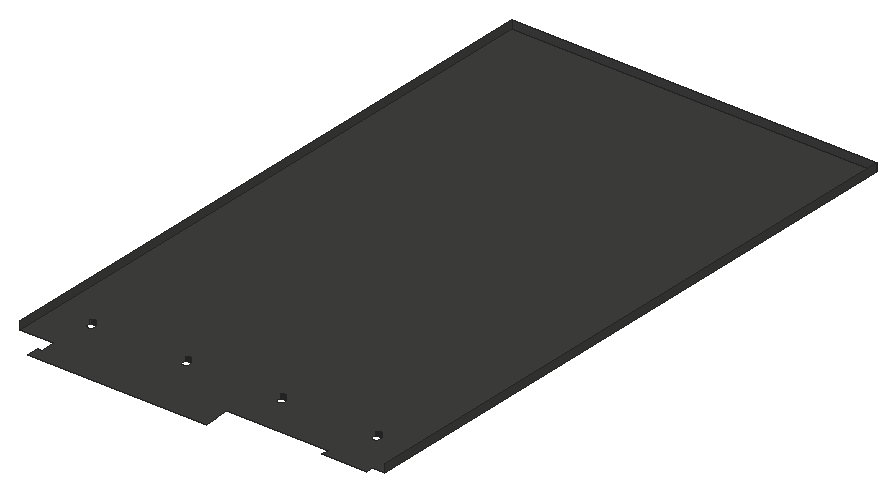
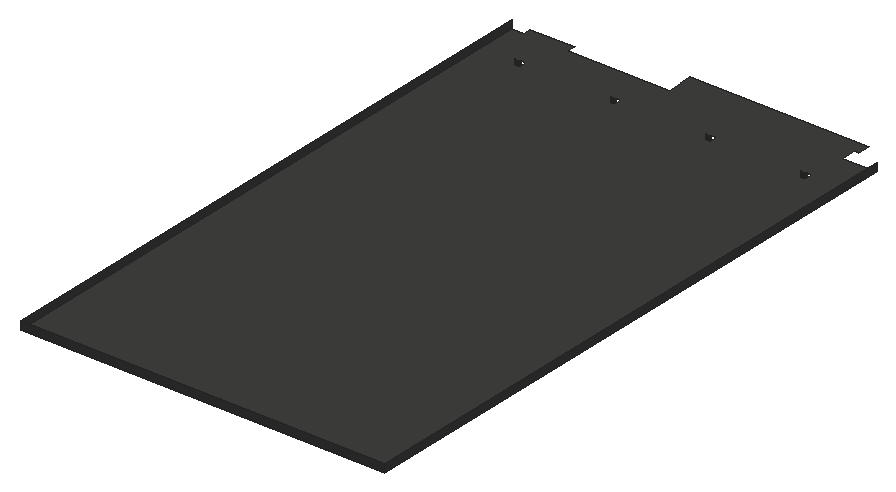
# SketchUp Ruby script. Lengths in inches.
U = 1.inch
M = Sketchup.active_model
def pt(a) = Geom::Point3d.new(a.map { |v| v * U })
def face(e, loops, mat)
  f = e.add_face(loops[0].map { |a| pt(a) })
  loops[1..].each { |l| e.add_face(l.map { |a| pt(a) }).erase! }
  f.material = f.back_material = mat if mat
  f
end
# faces: each face lists its corners as indices into pts; further lists are holes
def faces(e, pts, list, mat = nil) = list.each { |f| face(e, (f[0].is_a?(Array) ? f : [f]).map { |l| l.map { |i| pts[i] } }, mat) }
# xy, xz, yz: faces in a plane at the given z, y or x. An outline is a flat list of corners, or four numbers for a rectangle; further outlines are holes
def ring(l) = l.size == 4 ? [[l[0], l[1]], [l[2], l[1]], [l[2], l[3]], [l[0], l[3]]] : l.each_slice(2).to_a
def flat(e, list, mat, &to3) = list.each { |f| face(e, (f[0].is_a?(Array) ? f : [f]).map { |l| ring(l).map { |u, v| to3.(u, v) } }, mat) }
def xy(e, z, list, mat = nil) = flat(e, list, mat) { |x, y| [x, y, z] }
def xz(e, y, list, mat = nil) = flat(e, list, mat) { |x, z| [x, y, z] }
def yz(e, x, list, mat = nil) = flat(e, list, mat) { |y, z| [x, y, z] }
def lines(e, pts, list) = list.each { |a, b| e.add_line(pt(pts[a]), pt(pts[b])) }
# prism: a flat outline (further loops are holes) pulled along v
def prism(e, loops, v, mat = nil)
  f = face(e, loops, mat); d = Geom::Vector3d.new(v.map { |x| x * U })
  f.pushpull(f.normal.samedirection?(d) ? d.length : -d.length)
end
def box(e, o, s, mat = nil) = prism(e, [[o, [o[0] + s[0], o[1], o[2]], [o[0] + s[0], o[1] + s[1], o[2]], [o[0], o[1] + s[1], o[2]]]], [0, 0, s[2]], mat)
def at(x, y, z, deg = 0) = Geom::Transformation.translation(pt([x, y, z])) * Geom::Transformation.rotation(ORIGIN, Z_AXIS, deg.degrees)
def axes(o, x, y, z) = Geom::Transformation.new([*x, 0, *y, 0, *z, 0, *pt(o).to_a, 1])
def part(name) = M.definitions.add(name)
# library, detail: a bought-in or finely detailed component or shape, given as its bounding box
def library(name, o, s) = part(name).tap { |d| box(d.entities, o, s) }
def detail(e, o, s) = box(e.add_group.entities, o, s)
def put(e, d, t, mat = nil) = e.add_instance(d, t).tap { |i| i.material = mat if mat }
def group(e, t, mat = nil) = e.add_group.tap { |g| g.transformation = t; g.material = mat if mat }.entities
root = M.entities
M.materials.add("1448 AP 8253 RAVEN SONG").color = [64, 64, 63]
xy(root,372,[[[31.93,174,31.93,183,35.02,183,35.02,195,9.27,195,9.27,663,287.37,663,287.37,195,278.1,195,278.1,189,244.11,189,244.11,195,166.86,195,166.86,183,167.89,183,167.89,174],[257.03,221.5,257.35,221.5,257.43,221.51,257.5,221.52,257.74,221.55,257.8125,221.57,257.89,221.58,257.97,221.6,258.04,221.625,258.12,221.65,258.19,221.67,258.27,221.7,258.48,221.79,258.55,221.83,258.62,221.86,258.76,221.94,258.82,221.98,258.89,222.03,258.95,222.07,259.02,222.12,259.26,222.32,259.3125,222.38,259.37,222.43,259.57,222.67,259.62,222.74,259.66,222.8,259.71,222.87,259.75,222.93,259.83,223.07,259.86,223.14,259.9,223.21,259.99,223.42,260.02,223.5,260.04,223.57,260.07,223.65,260.09,223.72,260.11,223.8,260.14,223.95,260.16,224.11,260.17,224.1875,260.18,224.26,260.1875,224.34,260.1875,224.42,260.19,224.5,260.1875,224.58,260.1875,224.66,260.18,224.74,260.17,224.8125,260.16,224.89,260.14,225.05,260.11,225.2,260.09,225.28,260.07,225.35,260.04,225.43,260.02,225.5,259.99,225.58,259.9,225.79,259.86,225.86,259.83,225.93,259.75,226.07,259.71,226.13,259.66,226.2,259.62,226.26,259.57,226.33,259.37,226.57,259.3125,226.62,259.26,226.68,259.02,226.88,258.95,226.93,258.89,226.97,258.82,227.02,258.76,227.06,258.62,227.14,258.55,227.17,258.48,227.21,258.27,227.3,258.19,227.33,258.12,227.35,258.04,227.375,257.97,227.4,257.89,227.42,257.8125,227.43,257.74,227.45,257.5,227.48,257.43,227.49,257.35,227.5,257.03,227.5,256.95,227.49,256.8,227.47,256.64,227.45,256.57,227.43,256.49,227.42,256.41,227.4,256.34,227.375,256.26,227.35,256.1875,227.33,256.11,227.3,255.9,227.21,255.83,227.17,255.76,227.14,255.62,227.06,255.56,227.02,255.49,226.97,255.43,226.93,255.36,226.88,255.18,226.73,255.125,226.68,255.07,226.62,255.01,226.57,254.81,226.33,254.76,226.26,254.72,226.2,254.67,226.13,254.63,226.07,254.55,225.93,254.52,225.86,254.48,225.79,254.39,225.58,254.36,225.5,254.34,225.43,254.3125,225.35,254.29,225.28,254.27,225.2,254.26,225.125,254.24,225.05,254.22,224.89,254.21,224.8125,254.2,224.74,254.19,224.66,254.19,224.34,254.2,224.26,254.21,224.1875,254.22,224.11,254.24,223.95,254.26,223.875,254.27,223.8,254.29,223.72,254.3125,223.65,254.34,223.57,254.36,223.5,254.39,223.42,254.48,223.21,254.52,223.14,254.55,223.07,254.63,222.93,254.67,222.87,254.72,222.8,254.76,222.74,254.81,222.67,255.01,222.43,255.07,222.38,255.125,222.32,255.18,222.27,255.36,222.12,255.43,222.07,255.49,222.03,255.56,221.98,255.62,221.94,255.76,221.86,255.83,221.83,255.9,221.79,256.11,221.7,256.1875,221.67,256.26,221.65,256.34,221.625,256.41,221.6,256.49,221.58,256.57,221.57,256.64,221.55,256.8,221.53,256.95,221.51],[184.45,221.5,184.77,221.5,184.85,221.51,184.92,221.52,185.16,221.55,185.23,221.57,185.31,221.58,185.39,221.6,185.46,221.625,185.54,221.65,185.61,221.67,185.69,221.7,185.9,221.79,185.97,221.83,186.04,221.86,186.18,221.94,186.24,221.98,186.31,222.03,186.375,222.07,186.5,222.17,186.68,222.32,186.73,222.38,186.79,222.43,186.99,222.67,187.04,222.74,187.08,222.8,187.125,222.87,187.17,222.93,187.25,223.07,187.28,223.14,187.32,223.21,187.41,223.42,187.4375,223.5,187.46,223.57,187.49,223.65,187.51,223.72,187.53,223.8,187.54,223.875,187.56,223.95,187.58,224.11,187.59,224.1875,187.6,224.26,187.61,224.34,187.61,224.66,187.6,224.74,187.59,224.8125,187.58,224.89,187.56,225.05,187.54,225.125,187.53,225.2,187.51,225.28,187.49,225.35,187.46,225.43,187.4375,225.5,187.41,225.58,187.32,225.79,187.28,225.86,187.25,225.93,187.17,226.07,187.125,226.13,187.08,226.2,187.04,226.26,186.99,226.33,186.79,226.57,186.73,226.62,186.68,226.68,186.5,226.83,186.375,226.93,186.31,226.97,186.24,227.02,186.18,227.06,186.04,227.14,185.97,227.17,185.9,227.21,185.69,227.3,185.61,227.33,185.54,227.35,185.46,227.375,185.39,227.4,185.31,227.42,185.23,227.43,185.16,227.45,184.92,227.48,184.85,227.49,184.77,227.5,184.45,227.5,184.3,227.48,184.14,227.46,184.0625,227.45,183.99,227.43,183.91,227.42,183.83,227.4,183.76,227.375,183.68,227.35,183.61,227.33,183.53,227.3,183.32,227.21,183.25,227.17,183.18,227.14,183.04,227.06,182.98,227.02,182.91,226.97,182.85,226.93,182.78,226.88,182.54,226.68,182.49,226.62,182.43,226.57,182.23,226.33,182.18,226.26,182.14,226.2,182.09,226.13,182.05,226.07,181.97,225.93,181.9375,225.86,181.9,225.79,181.81,225.58,181.78,225.5,181.76,225.43,181.73,225.35,181.71,225.28,181.69,225.2,181.68,225.125,181.66,225.05,181.64,224.89,181.625,224.8125,181.62,224.74,181.61,224.66,181.61,224.34,181.62,224.26,181.625,224.1875,181.64,224.11,181.66,223.95,181.68,223.875,181.69,223.8,181.71,223.72,181.73,223.65,181.76,223.57,181.78,223.5,181.81,223.42,181.9,223.21,181.9375,223.14,181.97,223.07,182.05,222.93,182.09,222.87,182.14,222.8,182.18,222.74,182.23,222.67,182.43,222.43,182.49,222.38,182.54,222.32,182.78,222.12,182.85,222.07,182.91,222.03,182.98,221.98,183.04,221.94,183.18,221.86,183.25,221.83,183.32,221.79,183.53,221.7,183.61,221.67,183.68,221.65,183.76,221.625,183.83,221.6,183.91,221.58,183.99,221.57,184.0625,221.55,184.14,221.54,184.3,221.52],[39.29,221.5,39.61,221.5,39.69,221.51,39.76,221.52,40,221.55,40.07,221.57,40.15,221.58,40.23,221.6,40.3,221.625,40.38,221.65,40.45,221.67,40.53,221.7,40.74,221.79,40.8125,221.83,40.88,221.86,41.02,221.94,41.08,221.98,41.15,222.03,41.21,222.07,41.28,222.12,41.52,222.32,41.57,222.38,41.625,222.43,41.68,222.49,41.83,222.67,41.88,222.74,41.92,222.8,41.97,222.87,42.01,222.93,42.09,223.07,42.16,223.21,42.25,223.42,42.28,223.5,42.3,223.57,42.33,223.65,42.35,223.72,42.37,223.8,42.38,223.875,42.4,223.95,42.42,224.11,42.43,224.1875,42.44,224.26,42.45,224.34,42.45,224.66,42.44,224.74,42.43,224.8125,42.42,224.89,42.4,225.05,42.38,225.125,42.37,225.2,42.35,225.28,42.33,225.35,42.3,225.43,42.28,225.5,42.25,225.58,42.16,225.79,42.09,225.93,42.01,226.07,41.97,226.13,41.92,226.2,41.88,226.26,41.83,226.33,41.68,226.51,41.625,226.57,41.57,226.62,41.52,226.68,41.28,226.88,41.21,226.93,41.15,226.97,41.08,227.02,41.02,227.06,40.88,227.14,40.8125,227.17,40.74,227.21,40.53,227.3,40.45,227.33,40.38,227.35,40.3,227.375,40.23,227.4,40.15,227.42,40.07,227.43,40,227.45,39.76,227.48,39.69,227.49,39.61,227.5,39.29,227.5,39.21,227.49,39.14,227.48,38.9,227.45,38.83,227.43,38.75,227.42,38.67,227.4,38.6,227.375,38.52,227.35,38.45,227.33,38.3,227.27,38.16,227.21,38.09,227.17,38.02,227.14,37.88,227.06,37.82,227.02,37.75,226.97,37.6875,226.93,37.5,226.78,37.38,226.68,37.33,226.62,37.27,226.57,37.07,226.33,37.02,226.26,36.98,226.2,36.93,226.13,36.89,226.07,36.85,226,36.8125,225.93,36.78,225.86,36.74,225.79,36.65,225.58,36.62,225.5,36.6,225.43,36.57,225.35,36.55,225.28,36.53,225.2,36.52,225.125,36.5,225.05,36.48,224.89,36.47,224.8125,36.46,224.74,36.45,224.66,36.45,224.34,36.46,224.26,36.47,224.1875,36.48,224.11,36.5,223.95,36.52,223.875,36.53,223.8,36.55,223.72,36.57,223.65,36.6,223.57,36.62,223.5,36.65,223.42,36.74,223.21,36.78,223.14,36.8125,223.07,36.85,223,36.89,222.93,36.93,222.87,36.98,222.8,37.02,222.74,37.07,222.67,37.27,222.43,37.33,222.38,37.38,222.32,37.5,222.22,37.6875,222.07,37.75,222.03,37.82,221.98,37.88,221.94,38.02,221.86,38.09,221.83,38.16,221.79,38.3,221.73,38.45,221.67,38.52,221.65,38.6,221.625,38.67,221.6,38.75,221.58,38.83,221.57,38.9,221.55,39.14,221.52,39.21,221.51],[111.87,221.5,112.1875,221.5,112.27,221.51,112.34,221.52,112.58,221.55,112.65,221.57,112.73,221.58,112.81,221.6,112.88,221.625,112.96,221.65,113.03,221.67,113.11,221.7,113.32,221.79,113.39,221.83,113.46,221.86,113.6,221.94,113.66,221.98,113.73,222.03,113.79,222.07,113.86,222.12,114.1,222.32,114.15,222.38,114.21,222.43,114.26,222.49,114.3125,222.55,114.36,222.61,114.41,222.67,114.46,222.74,114.5,222.8,114.55,222.87,114.59,222.93,114.67,223.07,114.7,223.14,114.74,223.21,114.83,223.42,114.86,223.5,114.88,223.57,114.91,223.65,114.93,223.72,114.95,223.8,114.96,223.875,114.98,223.95,115,224.11,115.01,224.1875,115.02,224.26,115.03,224.34,115.03,224.66,115.02,224.74,115.01,224.8125,115,224.89,114.98,225.05,114.96,225.125,114.95,225.2,114.93,225.28,114.91,225.35,114.88,225.43,114.86,225.5,114.83,225.58,114.74,225.79,114.7,225.86,114.67,225.93,114.59,226.07,114.55,226.13,114.5,226.2,114.46,226.26,114.41,226.33,114.36,226.39,114.3125,226.45,114.26,226.51,114.21,226.57,114.15,226.62,114.1,226.68,113.86,226.88,113.79,226.93,113.73,226.97,113.66,227.02,113.6,227.06,113.46,227.14,113.39,227.17,113.32,227.21,113.11,227.3,113.03,227.33,112.96,227.35,112.88,227.375,112.81,227.4,112.73,227.42,112.65,227.43,112.58,227.45,112.34,227.48,112.27,227.49,112.1875,227.5,111.87,227.5,111.79,227.49,111.72,227.48,111.64,227.47,111.5625,227.46,111.48,227.45,111.41,227.43,111.33,227.42,111.25,227.4,111.18,227.375,111.1,227.35,111.03,227.33,110.95,227.3,110.74,227.21,110.67,227.17,110.6,227.14,110.46,227.06,110.4,227.02,110.33,226.97,110.27,226.93,110.2,226.88,109.96,226.68,109.91,226.62,109.85,226.57,109.65,226.33,109.6,226.26,109.56,226.2,109.51,226.13,109.47,226.07,109.39,225.93,109.36,225.86,109.32,225.79,109.23,225.58,109.2,225.5,109.18,225.43,109.15,225.35,109.13,225.28,109.11,225.2,109.1,225.125,109.08,225.05,109.06,224.89,109.05,224.8125,109.04,224.74,109.03,224.66,109.03,224.34,109.04,224.26,109.05,224.1875,109.06,224.11,109.08,223.95,109.1,223.875,109.11,223.8,109.13,223.72,109.15,223.65,109.18,223.57,109.2,223.5,109.23,223.42,109.32,223.21,109.36,223.14,109.39,223.07,109.47,222.93,109.51,222.87,109.56,222.8,109.6,222.74,109.65,222.67,109.85,222.43,109.91,222.38,109.96,222.32,110.2,222.12,110.27,222.07,110.33,222.03,110.4,221.98,110.46,221.94,110.6,221.86,110.67,221.83,110.74,221.79,110.95,221.7,111.03,221.67,111.1,221.65,111.18,221.625,111.25,221.6,111.33,221.58,111.41,221.57,111.48,221.55,111.5625,221.54,111.64,221.53,111.72,221.52,111.79,221.51]]],"1448 AP 8253 RAVEN SONG")
xz(root,227.5,[[39.29,372,39.37,375],[39.37,372,39.45,375],[39.45,372,39.53,375],[39.53,372,39.61,375],[111.87,372,111.95,375],
  [111.95,372,112.03,375],[112.03,372,112.11,375],[112.11,372,112.1875,375],[184.45,372,184.53,375],[184.53,372,184.61,375],
  [184.61,372,184.6875,375],[184.6875,372,184.77,375],[257.03,372,257.11,375],[257.11,372,257.19,375],[257.19,372,257.27,375],
  [257.27,372,257.35,375]],"1448 AP 8253 RAVEN SONG")
xz(root,663,[[9.27,372,287.37,378]],"1448 AP 8253 RAVEN SONG")
yz(root,9.27,[[195,372,663,378]],"1448 AP 8253 RAVEN SONG")
yz(root,287.37,[[195,372,663,378]],"1448 AP 8253 RAVEN SONG")
p = [[37.33,226.62,372],[37.38,226.68,372],[37.38,226.68,375],[37.33,226.62,375],[41.52,226.68,372],[41.57,226.62,372],
  [41.57,226.62,375],[41.52,226.68,375],[41.625,226.57,372],[41.625,226.57,375],[109.91,226.62,372],[109.96,226.68,372],
  [109.96,226.68,375],[109.91,226.62,375],[114.1,226.68,372],[114.15,226.62,372],[114.15,226.62,375],[114.1,226.68,375],
  [182.49,226.62,372],[182.54,226.68,372],[182.54,226.68,375],[182.49,226.62,375],[186.68,226.68,372],[186.73,226.62,372],
  [186.73,226.62,375],[186.68,226.68,375],[255.07,226.62,372],[255.125,226.68,372],[255.125,226.68,375],[255.07,226.62,375],
  [259.26,226.68,372],[259.3125,226.62,372],[259.3125,226.62,375],[259.26,226.68,375],[37.44,226.73,372],[37.44,226.73,375],
  [37.5,226.78,372],[37.5,226.78,375],[41.4,226.78,372],[41.46,226.73,372],[41.46,226.73,375],[41.4,226.78,375],
  [110.02,226.73,372],[110.02,226.73,375],[110.08,226.78,372],[110.08,226.78,375],[114.04,226.73,372],[114.04,226.73,375],
  [113.98,226.78,372],[113.98,226.78,375],[182.6,226.73,372],[182.6,226.73,375],[182.66,226.78,372],[182.66,226.78,375],
  [186.62,226.73,372],[186.62,226.73,375],[186.56,226.78,372],[186.56,226.78,375],[255.18,226.73,372],[255.18,226.73,375],
  [255.24,226.78,372],[255.24,226.78,375],[259.14,226.78,372],[259.2,226.73,372],[259.2,226.73,375],[259.14,226.78,375],
  [37.5625,226.83,372],[37.5625,226.83,375],[37.625,226.88,372],[37.625,226.88,375],[41.34,226.83,372],[41.34,226.83,375],
  [41.28,226.88,372],[41.28,226.88,375],[110.14,226.83,372],[110.14,226.83,375],[110.2,226.88,372],[110.2,226.88,375],
  [113.92,226.83,372],[113.92,226.83,375],[113.86,226.88,372],[113.86,226.88,375],[182.72,226.83,372],[182.72,226.83,375],
  [182.78,226.88,372],[182.78,226.88,375],[186.4375,226.88,372],[186.5,226.83,372],[186.5,226.83,375],[186.4375,226.88,375],
  [255.3,226.83,372],[255.3,226.83,375],[255.36,226.88,372],[255.36,226.88,375],[259.02,226.88,372],[259.08,226.83,372],
  [259.08,226.83,375],[259.02,226.88,375],[37.6875,226.93,372],[37.6875,226.93,375],[37.75,226.97,372],[37.75,226.97,375],
  [41.15,226.97,372],[41.21,226.93,372],[41.21,226.93,375],[41.15,226.97,375],[110.27,226.93,372],[110.27,226.93,375],
  [110.33,226.97,372],[110.33,226.97,375],[113.73,226.97,372],[113.79,226.93,372],[113.79,226.93,375],[113.73,226.97,375],
  [182.85,226.93,372],[182.85,226.93,375],[182.91,226.97,372],[182.91,226.97,375],[186.31,226.97,372],[186.375,226.93,372],
  [186.375,226.93,375],[186.31,226.97,375],[255.43,226.93,372],[255.43,226.93,375],[255.49,226.97,372],[255.49,226.97,375],
  [258.89,226.97,372],[258.95,226.93,372],[258.95,226.93,375],[258.89,226.97,375],[37.82,227.02,372],[37.82,227.02,375],
  [37.88,227.06,372],[37.88,227.06,375],[41.02,227.06,372],[41.08,227.02,372],[41.08,227.02,375],[41.02,227.06,375],
  [110.4,227.02,372],[110.4,227.02,375],[110.46,227.06,372],[110.46,227.06,375],[113.6,227.06,372],[113.66,227.02,372],
  [113.66,227.02,375],[113.6,227.06,375],[182.98,227.02,372],[182.98,227.02,375],[183.04,227.06,372],[183.04,227.06,375],
  [186.24,227.02,372],[186.24,227.02,375],[186.18,227.06,372],[186.18,227.06,375],[255.56,227.02,372],[255.56,227.02,375],
  [255.62,227.06,372],[255.62,227.06,375],[258.82,227.02,372],[258.82,227.02,375],[258.76,227.06,372],[258.76,227.06,375],
  [37.95,227.1,372],[37.95,227.1,375],[38.02,227.14,372],[38.02,227.14,375],[38.09,227.17,372],[38.09,227.17,375],
  [40.8125,227.17,372],[40.88,227.14,372],[40.88,227.14,375],[40.8125,227.17,375],[40.95,227.1,372],[40.95,227.1,375],
  [110.53,227.1,372],[110.53,227.1,375],[110.6,227.14,372],[110.6,227.14,375],[110.67,227.17,372],[110.67,227.17,375],
  [113.39,227.17,372],[113.46,227.14,372],[113.46,227.14,375],[113.39,227.17,375],[113.53,227.1,372],[113.53,227.1,375],
  [183.11,227.1,372],[183.11,227.1,375],[183.18,227.14,372],[183.18,227.14,375],[183.25,227.17,372],[183.25,227.17,375],
  [186.04,227.14,372],[186.11,227.1,372],[186.11,227.1,375],[186.04,227.14,375],[185.97,227.17,372],[185.97,227.17,375],
  [255.69,227.1,372],[255.69,227.1,375],[255.76,227.14,372],[255.76,227.14,375],[255.83,227.17,372],[255.83,227.17,375],
  [258.62,227.14,372],[258.69,227.1,372],[258.69,227.1,375],[258.62,227.14,375],[258.55,227.17,372],[258.55,227.17,375],
  [38.16,227.21,372],[38.16,227.21,375],[38.23,227.24,372],[38.23,227.24,375],[38.3,227.27,372],[38.3,227.27,375],
  [40.6,227.27,372],[40.67,227.24,372],[40.67,227.24,375],[40.6,227.27,375],[40.74,227.21,372],[40.74,227.21,375],
  [110.74,227.21,372],[110.74,227.21,375],[110.81,227.24,372],[110.81,227.24,375],[110.88,227.27,372],[110.88,227.27,375],
  [113.18,227.27,372],[113.25,227.24,372],[113.25,227.24,375],[113.18,227.27,375],[113.32,227.21,372],[113.32,227.21,375],
  [183.32,227.21,372],[183.32,227.21,375],[183.39,227.24,372],[183.39,227.24,375],[183.46,227.27,372],[183.46,227.27,375],
  [185.83,227.24,372],[185.9,227.21,372],[185.9,227.21,375],[185.83,227.24,375],[185.76,227.27,372],[185.76,227.27,375],
  [255.9,227.21,372],[255.9,227.21,375],[255.97,227.24,372],[255.97,227.24,375],[256.04,227.27,372],[256.04,227.27,375],
  [258.34,227.27,372],[258.41,227.24,372],[258.41,227.24,375],[258.34,227.27,375],[258.48,227.21,372],[258.48,227.21,375],
  [38.375,227.3,372],[38.375,227.3,375],[38.45,227.33,372],[38.45,227.33,375],[38.52,227.35,372],[38.52,227.35,375],
  [40.38,227.35,372],[40.45,227.33,372],[40.45,227.33,375],[40.38,227.35,375],[40.53,227.3,372],[40.53,227.3,375],
  [110.95,227.3,372],[110.95,227.3,375],[111.03,227.33,372],[111.03,227.33,375],[111.1,227.35,372],[111.1,227.35,375],
  [113.03,227.33,372],[113.11,227.3,372],[113.11,227.3,375],[113.03,227.33,375],[112.96,227.35,372],[112.96,227.35,375],
  [183.53,227.3,372],[183.53,227.3,375],[183.61,227.33,372],[183.61,227.33,375],[183.68,227.35,372],[183.68,227.35,375],
  [185.54,227.35,372],[185.61,227.33,372],[185.61,227.33,375],[185.54,227.35,375],[185.69,227.3,372],[185.69,227.3,375],
  [256.11,227.3,372],[256.11,227.3,375],[256.1875,227.33,372],[256.1875,227.33,375],[256.26,227.35,372],[256.26,227.35,375],
  [258.12,227.35,372],[258.19,227.33,372],[258.19,227.33,375],[258.12,227.35,375],[258.27,227.3,372],[258.27,227.3,375],
  [38.6,227.375,372],[38.6,227.375,375],[38.67,227.4,372],[38.67,227.4,375],[38.75,227.42,372],[38.75,227.42,375],
  [38.83,227.43,372],[38.83,227.43,375],[38.9,227.45,372],[38.9,227.45,375],[38.98,227.46,372],[38.98,227.46,375],
  [39.92,227.46,372],[40,227.45,372],[40,227.45,375],[39.92,227.46,375],[40.07,227.43,372],[40.07,227.43,375],
  [40.15,227.42,372],[40.15,227.42,375],[40.23,227.4,372],[40.3,227.375,372],[40.3,227.375,375],[40.23,227.4,375],
  [111.18,227.375,372],[111.18,227.375,375],[111.25,227.4,372],[111.25,227.4,375],[111.33,227.42,372],[111.33,227.42,375],
  [111.41,227.43,372],[111.41,227.43,375],[111.48,227.45,372],[111.48,227.45,375],[111.5625,227.46,372],[111.5625,227.46,375],
  [112.5,227.46,372],[112.58,227.45,372],[112.58,227.45,375],[112.5,227.46,375],[112.65,227.43,372],[112.65,227.43,375],
  [112.73,227.42,372],[112.81,227.4,372],[112.81,227.4,375],[112.73,227.42,375],[112.88,227.375,372],[112.88,227.375,375],
  [183.76,227.375,372],[183.76,227.375,375],[183.83,227.4,372],[183.83,227.4,375],[183.91,227.42,372],[183.91,227.42,375],
  [183.99,227.43,372],[183.99,227.43,375],[184.0625,227.45,372],[184.0625,227.45,375],[184.14,227.46,372],[184.14,227.46,375],
  [185.08,227.46,372],[185.16,227.45,372],[185.16,227.45,375],[185.08,227.46,375],[185.23,227.43,372],[185.31,227.42,372],
  [185.31,227.42,375],[185.23,227.43,375],[185.39,227.4,372],[185.39,227.4,375],[185.46,227.375,372],[185.46,227.375,375],
  [256.34,227.375,372],[256.34,227.375,375],[256.41,227.4,372],[256.41,227.4,375],[256.49,227.42,372],[256.49,227.42,375],
  [256.57,227.43,372],[256.57,227.43,375],[256.64,227.45,372],[256.64,227.45,375],[256.72,227.46,372],[256.72,227.46,375],
  [257.74,227.45,372],[257.8125,227.43,372],[257.8125,227.43,375],[257.74,227.45,375],[257.66,227.46,372],[257.66,227.46,375],
  [257.89,227.42,372],[257.89,227.42,375],[257.97,227.4,372],[257.97,227.4,375],[258.04,227.375,372],[258.04,227.375,375],
  [39.06,227.47,372],[39.06,227.47,375],[39.14,227.48,372],[39.14,227.48,375],[39.21,227.49,372],[39.21,227.49,375],
  [39.29,227.5,372],[39.29,227.5,375],[39.61,227.5,372],[39.69,227.49,372],[39.69,227.49,375],[39.61,227.5,375],
  [39.76,227.48,372],[39.76,227.48,375],[39.84,227.47,372],[39.84,227.47,375],[111.64,227.47,372],[111.64,227.47,375],
  [111.72,227.48,372],[111.72,227.48,375],[111.79,227.49,372],[111.79,227.49,375],[111.87,227.5,372],[111.87,227.5,375],
  [112.1875,227.5,372],[112.27,227.49,372],[112.27,227.49,375],[112.1875,227.5,375],[112.34,227.48,372],[112.42,227.47,372],
  [112.42,227.47,375],[112.34,227.48,375],[184.22,227.47,372],[184.22,227.47,375],[184.3,227.48,372],[184.3,227.48,375],
  [184.375,227.49,372],[184.375,227.49,375],[184.45,227.5,372],[184.45,227.5,375],[184.85,227.49,372],[184.92,227.48,372],
  [184.92,227.48,375],[184.85,227.49,375],[184.77,227.5,372],[184.77,227.5,375],[185,227.47,372],[185,227.47,375],
  [256.8,227.47,372],[256.8,227.47,375],[256.875,227.48,372],[256.875,227.48,375],[256.95,227.49,372],[256.95,227.49,375],
  [257.03,227.5,372],[257.03,227.5,375],[257.35,227.5,372],[257.43,227.49,372],[257.43,227.49,375],[257.35,227.5,375],
  [257.5,227.48,372],[257.5,227.48,375],[257.58,227.47,372],[257.58,227.47,375]]
faces(root,p,[[0,1,2,3],[4,5,6,7],[5,8,9,6],[10,11,12,13],[14,15,16,17],[18,19,20,21],[22,23,24,25],[26,27,28,29],
  [30,31,32,33],[1,34,35,2],[34,36,37,35],[38,39,40,41],[39,4,7,40],[11,42,43,12],[42,44,45,43],[46,14,17,47],
  [48,46,47,49],[19,50,51,20],[50,52,53,51],[54,22,25,55],[56,54,55,57],[27,58,59,28],[58,60,61,59],[62,63,64,65],
  [63,30,33,64],[36,66,67,37],[66,68,69,67],[70,38,41,71],[72,70,71,73],[44,74,75,45],[74,76,77,75],[78,48,49,79],
  [80,78,79,81],[52,82,83,53],[82,84,85,83],[86,87,88,89],[87,56,57,88],[60,90,91,61],[90,92,93,91],[94,95,96,97],
  [95,62,65,96],[68,98,99,69],[98,100,101,99],[102,103,104,105],[103,72,73,104],[76,106,107,77],[106,108,109,107],[110,111,112,113],
  [111,80,81,112],[84,114,115,85],[114,116,117,115],[118,119,120,121],[119,86,89,120],[92,122,123,93],[122,124,125,123],[126,127,128,129],
  [127,94,97,128],[100,130,131,101],[130,132,133,131],[134,135,136,137],[135,102,105,136],[108,138,139,109],[138,140,141,139],[142,143,144,145],
  [143,110,113,144],[116,146,147,117],[146,148,149,147],[150,118,121,151],[152,150,151,153],[124,154,155,125],[154,156,157,155],[158,126,129,159],
  [160,158,159,161],[132,162,163,133],[162,164,165,163],[164,166,167,165],[168,169,170,171],[172,134,137,173],[169,172,173,170],[140,174,175,141],
  [174,176,177,175],[176,178,179,177],[180,181,182,183],[184,142,145,185],[181,184,185,182],[148,186,187,149],[186,188,189,187],[188,190,191,189],
  [192,193,194,195],[196,192,195,197],[193,152,153,194],[156,198,199,157],[198,200,201,199],[200,202,203,201],[204,205,206,207],[208,204,207,209],
  [205,160,161,206],[166,210,211,167],[210,212,213,211],[212,214,215,213],[216,217,218,219],[220,168,171,221],[217,220,221,218],[178,222,223,179],
  [222,224,225,223],[224,226,227,225],[228,229,230,231],[232,180,183,233],[229,232,233,230],[190,234,235,191],[234,236,237,235],[236,238,239,237],
  [240,241,242,243],[244,240,243,245],[241,196,197,242],[202,246,247,203],[246,248,249,247],[248,250,251,249],[252,253,254,255],[253,256,257,254],
  [256,208,209,257],[214,258,259,215],[258,260,261,259],[260,262,263,261],[264,265,266,267],[268,216,219,269],[265,268,269,266],[226,270,271,227],
  [270,272,273,271],[272,274,275,273],[276,277,278,279],[280,276,279,281],[277,228,231,278],[238,282,283,239],[282,284,285,283],[284,286,287,285],
  [288,289,290,291],[289,292,293,290],[292,244,245,293],[250,294,295,251],[294,296,297,295],[296,298,299,297],[300,301,302,303],[301,304,305,302],
  [304,252,255,305],[262,306,307,263],[306,308,309,307],[308,310,311,309],[310,312,313,311],[312,314,315,313],[314,316,317,315],[318,319,320,321],
  [319,322,323,320],[322,324,325,323],[326,327,328,329],[324,326,329,325],[327,264,267,328],[274,330,331,275],[330,332,333,331],[332,334,335,333],
  [334,336,337,335],[336,338,339,337],[338,340,341,339],[342,343,344,345],[343,346,347,344],[348,349,350,351],[346,348,351,347],[349,352,353,350],
  [352,280,281,353],[286,354,355,287],[354,356,357,355],[356,358,359,357],[358,360,361,359],[360,362,363,361],[362,364,365,363],[366,367,368,369],
  [370,371,372,373],[367,370,373,368],[371,374,375,372],[374,376,377,375],[376,288,291,377],[298,378,379,299],[378,380,381,379],[380,382,383,381],
  [382,384,385,383],[384,386,387,385],[386,388,389,387],[390,391,392,393],[394,390,393,395],[391,396,397,392],[396,398,399,397],[400,300,303,401],
  [398,400,401,399],[316,402,403,317],[402,404,405,403],[404,406,407,405],[406,408,409,407],[410,411,412,413],[411,414,415,412],[416,318,321,417],
  [414,416,417,415],[340,418,419,341],[418,420,421,419],[420,422,423,421],[422,424,425,423],[426,427,428,429],[430,431,432,433],[427,430,433,428],
  [431,342,345,432],[364,434,435,365],[434,436,437,435],[436,438,439,437],[438,440,441,439],[442,443,444,445],[446,442,445,447],[443,448,449,444],
  [448,366,369,449],[388,450,451,389],[450,452,453,451],[452,454,455,453],[454,456,457,455],[458,459,460,461],[459,462,463,460],[462,464,465,463],
  [464,394,395,465]],"1448 AP 8253 RAVEN SONG")
